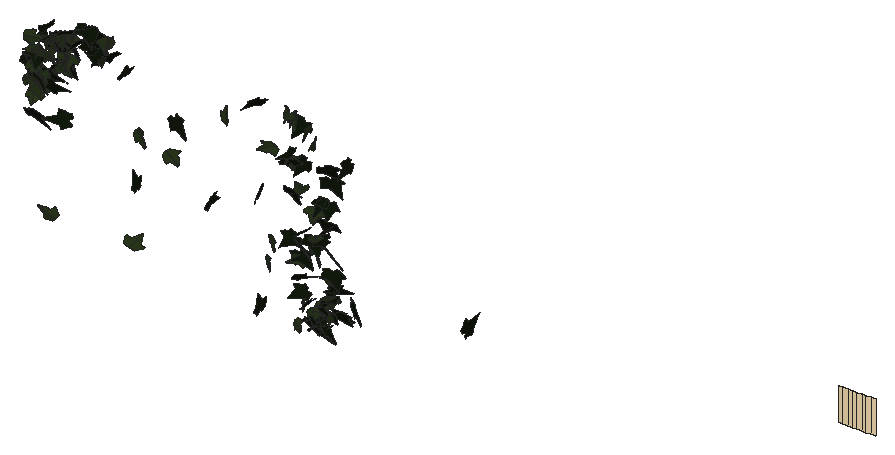
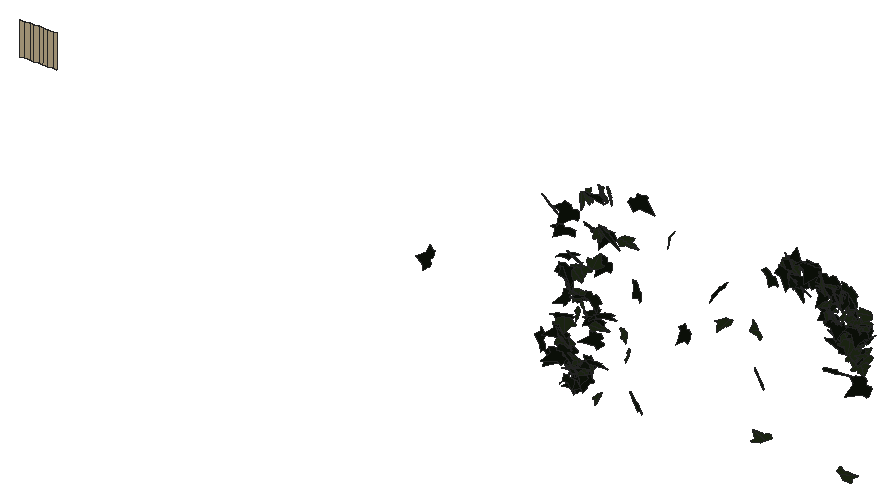
# SketchUp Ruby script. Lengths in inches.
U = 1.inch
M = Sketchup.active_model
def pt(a) = Geom::Point3d.new(a.map { |v| v * U })
def face(e, loops, mat)
  f = e.add_face(loops[0].map { |a| pt(a) })
  loops[1..].each { |l| e.add_face(l.map { |a| pt(a) }).erase! }
  f.material = f.back_material = mat if mat
  f
end
# faces: each face lists its corners as indices into pts; further lists are holes
def faces(e, pts, list, mat = nil) = list.each { |f| face(e, (f[0].is_a?(Array) ? f : [f]).map { |l| l.map { |i| pts[i] } }, mat) }
# xy, xz, yz: faces in a plane at the given z, y or x. An outline is a flat list of corners, or four numbers for a rectangle; further outlines are holes
def ring(l) = l.size == 4 ? [[l[0], l[1]], [l[2], l[1]], [l[2], l[3]], [l[0], l[3]]] : l.each_slice(2).to_a
def flat(e, list, mat, &to3) = list.each { |f| face(e, (f[0].is_a?(Array) ? f : [f]).map { |l| ring(l).map { |u, v| to3.(u, v) } }, mat) }
def xy(e, z, list, mat = nil) = flat(e, list, mat) { |x, y| [x, y, z] }
def xz(e, y, list, mat = nil) = flat(e, list, mat) { |x, z| [x, y, z] }
def yz(e, x, list, mat = nil) = flat(e, list, mat) { |y, z| [x, y, z] }
def lines(e, pts, list) = list.each { |a, b| e.add_line(pt(pts[a]), pt(pts[b])) }
# prism: a flat outline (further loops are holes) pulled along v
def prism(e, loops, v, mat = nil)
  f = face(e, loops, mat); d = Geom::Vector3d.new(v.map { |x| x * U })
  f.pushpull(f.normal.samedirection?(d) ? d.length : -d.length)
end
def box(e, o, s, mat = nil) = prism(e, [[o, [o[0] + s[0], o[1], o[2]], [o[0] + s[0], o[1] + s[1], o[2]], [o[0], o[1] + s[1], o[2]]]], [0, 0, s[2]], mat)
def at(x, y, z, deg = 0) = Geom::Transformation.translation(pt([x, y, z])) * Geom::Transformation.rotation(ORIGIN, Z_AXIS, deg.degrees)
def axes(o, x, y, z) = Geom::Transformation.new([*x, 0, *y, 0, *z, 0, *pt(o).to_a, 1])
def part(name) = M.definitions.add(name)
# library, detail: a bought-in or finely detailed component or shape, given as its bounding box
def library(name, o, s) = part(name).tap { |d| box(d.entities, o, s) }
def detail(e, o, s) = box(e.add_group.entities, o, s)
def put(e, d, t, mat = nil) = e.add_instance(d, t).tap { |i| i.material = mat if mat }
def group(e, t, mat = nil) = e.add_group.tap { |g| g.transformation = t; g.material = mat if mat }.entities
root = M.entities
M.materials.add("1026 AP 7946 SUNNY SIDE UP").color = [254, 231, 186]
M.materials.add("efeu1").color = [18, 25, 13]
M.materials.add("efeu2").color = [43, 57, 29]
c1 = part("ivyleaf_9")
p = [[1.54,2.16,1.25],[1.36,2.04,1.19],[-0.21,0.99,0.68],[-0.71,1.11,0.82],[-0.85,0.86,0.67],[-0.8,0.17,0.21],
  [-0.9,-0.01,0.1],[-0.67,-0.16,-0.02],[-0.08,-0.08,-0.05],[-0.03,-0.6,-0.4],[0.65,-0.88,-0.66],[0.83,-0.6,-0.49],
  [1.29,-0.42,-0.43],[1.8125,-0.07,-0.26],[1.21,0.44,0.15]]
faces(c1.entities,p,[[0,1,2,3,4,5,6,7,8,9,10,11,12,13,14]],"efeu1")
c2 = part("ivyleaf_10")
p = [[0,0.5,-0.03],[-0.0625,2.02,-0.43],[-0.19,2.01,-0.46],[-0.54,1.05,-0.29],[-0.52,0.625,-0.18],[-0.83,0.76,-0.28],
  [-1.16,0.64,-0.33],[-1.15,0.33,-0.24],[-0.77,-0.39,0.02],[-0.3,-0.51,0.16],[0.04,-0.48,0.23],[-0.02,2.01,-0.4375],
  [-0.06,2.01,-0.43],[0.04,-0.49,0.23],[0.67,-0.49,0.14],[1.38,0.36,-0.2],[1.375,0.51,-0.24],[0.81,0.65,-0.19],
  [0.62,0.59,-0.15],[0.6,1.09,-0.28],[0.5,1.23,-0.31]]
faces(c2.entities,p,[[0,1,2,3,4,5,6,7,8,9,10],[11,12,0,13,14,15,16,17,18,19,20]],"efeu2")
xz(root,213,[[177,274,177.27,276]],"1026 AP 7946 SUNNY SIDE UP")
xz(root,213.01,[[177.54,274,177.82,276]],"1026 AP 7946 SUNNY SIDE UP")
p = [[177.54,213.01,276],[177.27,213,276],[177.27,213,274],[177.54,213.01,274],[178.09,213.02,276],[177.82,213.01,276],
  [177.82,213.01,274],[178.09,213.02,274],[178.36,213.04,276],[178.36,213.04,274],[178.63,213.05,276],[178.63,213.05,274],
  [178.9,213.07,276],[178.9,213.07,274],[179.18,213.09,276],[179.18,213.09,274]]
faces(root,p,[[0,1,2,3],[4,5,6,7],[8,4,7,9],[10,8,9,11],[12,10,11,13],[14,12,13,15]],"1026 AP 7946 SUNNY SIDE UP")
put(root,c1,axes([127.72,212.82,276.75],[0.3772,-0.17588,-0.0113],[-0.03293,-0.01175,-0.30568],[0.27503,0.23981,-0.0211]),"1026 AP 7946 SUNNY SIDE UP")
put(root,c1,axes([127.84,212.98,276.51],[-0.03313,-0.29209,0.03896],[-0.00412,-0.03939,-0.30192],[0.46344,-0.02123,0.0001]),"1026 AP 7946 SUNNY SIDE UP")
put(root,c2,axes([127.84,212.9375,275.58],[0.19907,0.21946,0.15502],[0.10288,0.13443,-0.26006],[-0.40443,0.14222,0.01015]),"1026 AP 7946 SUNNY SIDE UP")
put(root,c2,axes([128.36,212.99,275.375],[-0.19765,-0.16137,-0.29884],[-0.3084,-0.21293,0.209],[-0.41954,0.23255,-0.01284]),"1026 AP 7946 SUNNY SIDE UP")
put(root,c2,axes([128.24,212.89,277.32],[-0.28047,-0.24117,0.03904],[0.03255,-0.06335,-0.30437],[0.38282,-0.1713,0.05448]),"1026 AP 7946 SUNNY SIDE UP")
put(root,c2,axes([127.87,212.87,277.85],[0.01117,-0.04427,-0.31213],[0.47775,0.03654,0.00205],[0.05643,-0.3006,0.0444]),"1026 AP 7946 SUNNY SIDE UP")
put(root,c2,axes([128.22,212.84,274.9],[0.26575,0.23024,-0.07491],[-0.06573,-0.06114,-0.29458],[-0.37456,0.17408,-0.00145]),"1026 AP 7946 SUNNY SIDE UP")
put(root,c1,axes([128.29,212.93,276.88],[0.24041,0.25089,-0.02975],[-0.00445,-0.03372,-0.30247],[-0.39734,0.15218,-0.01462]),"1026 AP 7946 SUNNY SIDE UP")
put(root,c2,axes([128.28,212.81,276.48],[0.30804,0.21571,-0.04422],[-0.04426,-0.03407,-0.30038],[-0.34337,0.19791,-0.00095]),"1026 AP 7946 SUNNY SIDE UP")
put(root,c1,axes([128.06,213.05,275.61],[0.33056,-0.19766,0.04801],[0.03066,-0.04874,-0.2967],[0.31826,0.21,-0.02129]),"1026 AP 7946 SUNNY SIDE UP")
put(root,c1,axes([128.11,212.73,273.87],[0.55453,-0.02015,0.01727],[0.0234,-0.03414,-0.36249],[0.03408,0.35141,-0.03215]),"1026 AP 7946 SUNNY SIDE UP")
put(root,c2,axes([128.41,212.91,277.33],[0.1914,-0.27526,-0.02861],[0.00493,0.03001,-0.30951],[0.43476,0.12084,0.01611]),"1026 AP 7946 SUNNY SIDE UP")
put(root,c2,axes([128.42,212.87,277.14],[-0.43618,-0.11328,-0.0391],[0.07091,-0.01219,-0.30739],[0.17361,-0.27963,0.02733]),"1026 AP 7946 SUNNY SIDE UP")
put(root,c1,axes([128.39,212.96,277.1],[-0.24385,-0.25558,-0.01952],[0.07625,-0.00921,-0.30434],[0.39554,-0.15579,0.04664]),"1026 AP 7946 SUNNY SIDE UP")
put(root,c2,axes([128.62,212.82,275.27],[-0.33885,-0.20376,-0.00949],[0.07116,-0.03636,-0.29995],[0.31264,-0.21256,0.05798]),"1026 AP 7946 SUNNY SIDE UP")
put(root,c1,axes([128.42,212.95,275.92],[0.10873,-0.28118,0.05193],[0.00159,-0.05327,-0.29838],[0.44963,0.06819,-0.0115]),"1026 AP 7946 SUNNY SIDE UP")
put(root,c2,axes([128.78,212.875,277.31],[-0.39148,0.15558,0.05274],[-0.08242,0.01087,-0.3018],[-0.24354,-0.25377,0.01736]),"1026 AP 7946 SUNNY SIDE UP")
put(root,c1,axes([128.98,212.83,278.2],[0.09419,-0.01024,-0.31194],[-0.47602,0.0086,-0.06196],[0.01639,0.30849,-0.00682]),"1026 AP 7946 SUNNY SIDE UP")
put(root,c2,axes([128.78,213.05,276.11],[-0.31893,-0.20553,-0.05828],[0.07414,0.03126,-0.29707],[0.32641,-0.20792,0.01052]),"1026 AP 7946 SUNNY SIDE UP")
put(root,c2,axes([128.56,212.9,275.94],[-0.09362,-0.03822,-0.29694],[0.4441,0.06135,-0.06818],[0.10716,-0.28764,0.02312]),"1026 AP 7946 SUNNY SIDE UP")
put(root,c1,axes([129.11,212.68,278.77],[-0.08346,0.29508,0.10232],[-0.08524,0.08876,-0.30614],[-0.48124,-0.06689,0.03648]),"1026 AP 7946 SUNNY SIDE UP")
put(root,c2,axes([129.14,212.74,278.06],[-0.39491,0.13264,0.11658],[-0.17931,0.0234,-0.2908],[-0.20636,-0.27416,0.02959]),"1026 AP 7946 SUNNY SIDE UP")
put(root,c2,axes([129.38,212.8,268.59],[0.20641,0.05303,0.27768],[-0.41919,-0.0461,0.14299],[0.10227,-0.29597,0.02565]),"1026 AP 7946 SUNNY SIDE UP")
put(root,c2,axes([129.125,212.91,276.26],[-0.16047,-0.26226,0.09568],[0.04108,-0.10905,-0.28376],[0.43633,-0.08619,0.0619]),"1026 AP 7946 SUNNY SIDE UP")
put(root,c1,axes([129.25,212.66,278.4],[0.13481,0.28631,0.09483],[0.04095,0.08659,-0.30739],[-0.47033,0.08961,0.00042]),"1026 AP 7946 SUNNY SIDE UP")
put(root,c2,axes([129.26,212.8,277.45],[-0.09505,0.29159,0.03706],[-0.03996,0.02971,-0.30599],[-0.45992,-0.06284,0.01893]),"1026 AP 7946 SUNNY SIDE UP")
put(root,c2,axes([129.34,212.88,278.39],[0.05604,-0.30396,-0.03565],[-0.00996,0.03236,-0.31509],[0.48064,0.03611,-0.00237]),"1026 AP 7946 SUNNY SIDE UP")
put(root,c1,axes([128.95,212.89,276.16],[0.24432,-0.06917,0.25192],[0.32008,-0.13848,-0.17413],[0.24023,0.25487,-0.0242]),"1026 AP 7946 SUNNY SIDE UP")
put(root,c2,axes([129.45,212.8,278.22],[-0.1584,0.28264,0.06675],[-0.06656,0.05181,-0.30798],[-0.4505,-0.10703,0.02203]),"1026 AP 7946 SUNNY SIDE UP")
put(root,c1,axes([129.09,212.83,275.61],[0.21776,-0.03194,0.26995],[0.37102,-0.11815,-0.1439],[0.18675,0.27199,-0.02889]),"1026 AP 7946 SUNNY SIDE UP")
put(root,c1,axes([129.58,212.93,276.82],[0.15077,0.28234,0.00082],[0.02255,-0.00573,-0.3068],[-0.44338,0.09572,-0.01533]),"1026 AP 7946 SUNNY SIDE UP")
put(root,c1,axes([130.12,212.88,278.02],[-0.23549,0.20348,0.17609],[-0.17196,0.13017,-0.25935],[-0.37956,-0.18522,0.00825]),"1026 AP 7946 SUNNY SIDE UP")
put(root,c1,axes([130.2,212.88,274.03],[-0.37111,0.06562,0.1874],[-0.30267,-0.05859,-0.23634],[-0.02267,-0.29193,0.08769]),"1026 AP 7946 SUNNY SIDE UP")
put(root,c1,axes([129.58,212.98,277.93],[0.31187,-0.22627,-0.02112],[0.01989,0.03647,-0.30784],[0.35651,0.1959,0.03564]),"1026 AP 7946 SUNNY SIDE UP")
put(root,c2,axes([129.84,212.91,278.43],[0.19956,-0.26697,0.08135],[0.0486,-0.07442,-0.30493],[0.43574,0.13057,-0.00325]),"1026 AP 7946 SUNNY SIDE UP")
put(root,c1,axes([129.51,212.9,278.18],[0.1997,-0.06727,0.2771],[0.32797,-0.17237,-0.14667],[0.28812,0.24284,-0.0251]),"1026 AP 7946 SUNNY SIDE UP")
put(root,c2,axes([129.78,212.9,277],[0.19238,-0.19906,-0.19635],[0.18736,-0.14846,0.23909],[-0.38938,-0.16978,0.01803]),"1026 AP 7946 SUNNY SIDE UP")
put(root,c2,axes([129.99,212.83,277.72],[0.12334,0.28494,0.05984],[-0.01354,0.06075,-0.3031],[-0.45655,0.07518,0.02516]),"1026 AP 7946 SUNNY SIDE UP")
put(root,c2,axes([129.74,212.89,276.88],[0.24954,0.01367,0.26287],[0.39819,0.03109,-0.16384],[-0.05285,0.29881,0.00679]),"1026 AP 7946 SUNNY SIDE UP")
put(root,c2,axes([130.15,212.88,278.51],[-0.16568,-0.28228,0.06208],[0.006,-0.0672,-0.30958],[0.45434,-0.10204,0.02673]),"1026 AP 7946 SUNNY SIDE UP")
put(root,c2,axes([130,213.03,277.07],[0.44773,-0.07765,0.04491],[0.07586,0.01002,-0.30314],[0.11809,0.28795,0.02447]),"1026 AP 7946 SUNNY SIDE UP")
put(root,c2,axes([130.15,212.79,277.42],[0.10909,-0.27345,-0.10525],[-0.00688,0.10244,-0.28932],[0.4581,0.06665,0.02072]),"1026 AP 7946 SUNNY SIDE UP")
put(root,c2,axes([130.16,212.81,278.57],[-0.37367,-0.18679,-0.06185],[0.11683,-0.00016,-0.30789],[0.28498,-0.24485,0.04512]),"1026 AP 7946 SUNNY SIDE UP")
put(root,c1,axes([130.28,212.73,278.94],[0.15874,0.28628,-0.06325],[-0.05359,-0.05474,-0.31273],[-0.4578,0.10567,0.01468]),"1026 AP 7946 SUNNY SIDE UP")
put(root,c2,axes([130.3,212.91,277.53],[-0.47357,-0.01469,0.02581],[-0.02733,-0.11885,-0.2868],[0.03673,-0.27787,0.11937]),"1026 AP 7946 SUNNY SIDE UP")
put(root,c1,axes([129.99,212.96,277.1875],[-0.14435,-0.07678,-0.28345],[0.38085,0.13143,-0.12046],[0.23688,-0.2581,0.02095]),"1026 AP 7946 SUNNY SIDE UP")
put(root,c2,axes([130.17,212.96,278.64],[0.40143,0.16201,0.01092],[0.02784,-0.00987,-0.31101],[-0.25367,0.25529,-0.01686]),"1026 AP 7946 SUNNY SIDE UP")
put(root,c1,axes([130.41,212.89,278.2],[0.40251,-0.09391,-0.14249],[-0.21722,0.02192,-0.27968],[0.14683,0.28988,-0.02313]),"1026 AP 7946 SUNNY SIDE UP")
put(root,c2,axes([130.42,212.98,278.62],[0.17879,-0.27689,-0.05731],[0.04385,-0.04696,0.30799],[-0.44143,-0.11681,0.00738]),"1026 AP 7946 SUNNY SIDE UP")
put(root,c1,axes([131.08,212.86,278.6875],[-0.16575,0.2283,-0.17618],[0.03456,-0.17664,-0.25597],[-0.44842,-0.098,0.04539]),"1026 AP 7946 SUNNY SIDE UP")
put(root,c1,axes([131.1,212.88,279.29],[0.26798,0.2545,0.05896],[0.07289,0.03598,-0.31477],[-0.40314,0.17568,-0.01772]),"1026 AP 7946 SUNNY SIDE UP")
put(root,c1,axes([131.42,212.96,279.42],[-0.23596,-0.22658,-0.15069],[0.1514,0.10978,-0.27876],[0.39495,-0.17745,0.01683]),"1026 AP 7946 SUNNY SIDE UP")
put(root,c1,axes([131.46,212.9,278.32],[-0.06059,0.01459,0.31302],[0.45376,0.09835,0.03342],[-0.15086,0.28997,-0.02519]),"1026 AP 7946 SUNNY SIDE UP")
put(root,c1,axes([132.22,212.82,278.08],[-0.19198,0.20042,0.20833],[-0.19808,0.15792,-0.24002],[-0.40006,-0.17436,0.01887]),"1026 AP 7946 SUNNY SIDE UP")
put(root,c1,axes([132.26,212.8125,278.08],[-0.12065,0.29944,-0.0002],[-0.00639,-0.00299,-0.31843],[-0.47081,-0.0767,0.00437]),"1026 AP 7946 SUNNY SIDE UP")
put(root,c2,axes([132.42,213.01,279.125],[-0.3998,0.01628,0.17805],[-0.26533,-0.0945,-0.24726],[0.06347,-0.2925,0.0879]),"1026 AP 7946 SUNNY SIDE UP")
put(root,c1,axes([132.29,212.88,278.93],[0.25728,0.14098,0.22892],[-0.29182,-0.12237,0.22084],[0.29187,-0.24662,0.01901]),"1026 AP 7946 SUNNY SIDE UP")
put(root,c2,axes([132.55,212.8125,278.31],[0.05576,-0.30783,-0.01434],[-0.00173,0.01212,-0.31915],[0.4844,0.03548,0.00051]),"1026 AP 7946 SUNNY SIDE UP")
put(root,c2,axes([132.6,212.89,279.23],[-0.27559,-0.25118,0.04992],[0.02558,-0.07125,-0.31111],[0.40186,-0.16772,0.05404]),"1026 AP 7946 SUNNY SIDE UP")
put(root,c1,axes([132.76,212.81,278.48],[0.12967,0.29952,-0.00782],[0.00703,-0.01087,-0.32003],[-0.47115,0.08228,-0.00692]),"1026 AP 7946 SUNNY SIDE UP")
put(root,c2,axes([132.64,212.9,279.24],[0.34883,-0.21175,0.047],[0.06762,-0.0227,-0.31578],[0.33422,0.22559,0.01484]),"1026 AP 7946 SUNNY SIDE UP")
put(root,c1,axes([133.78,212.73,277.83],[0.08933,0.21082,0.23128],[-0.03226,0.22919,-0.21619],[-0.4818,0.02374,0.05736]),"1026 AP 7946 SUNNY SIDE UP")
put(root,c1,axes([134.53,212.75,271.98],[-0.01133,0.08904,0.33242],[-0.08047,0.31815,-0.0899],[-0.51937,-0.05124,0.00668]),"1026 AP 7946 SUNNY SIDE UP")
put(root,c2,axes([134.28,212.71,268.79],[0.32912,0.13796,-0.20637],[0.23478,0.13704,0.25775],[0.3032,-0.25588,0.02442]),"1026 AP 7946 SUNNY SIDE UP")
put(root,c2,axes([134.41,213.02,274.77],[0.24533,-0.09537,0.29509],[0.41343,-0.11677,-0.18792],[0.23493,0.30508,0.02254]),"1026 AP 7946 SUNNY SIDE UP")
put(root,c2,axes([136.46,212.79,274.44],[0.14789,0.27129,0.16515],[0.11423,0.14247,-0.2943],[-0.48088,0.11728,-0.01912]),"1026 AP 7946 SUNNY SIDE UP")
put(root,c1,axes([136.64,213.02,276.3],[0.17637,-0.28511,-0.17208],[-0.12822,0.14529,-0.31411],[0.50218,0.13723,-0.01977]),"1026 AP 7946 SUNNY SIDE UP")
put(root,c1,axes([139.11,212.58,272.91],[-0.06118,0.08433,-0.33385],[-0.2875,0.26854,0.09604],[0.44198,0.18635,0.01626]),"1026 AP 7946 SUNNY SIDE UP")
put(root,c2,axes([140,212.625,277.63],[-0.00525,0.19291,-0.28334],[-0.0527,0.27458,0.19965],[0.52702,0.02938,0.01714]),"1026 AP 7946 SUNNY SIDE UP")
put(root,c1,axes([141.85,212.87,279.23],[-0.13009,0.18799,-0.24589],[-0.03412,-0.25144,-0.19687],[-0.47784,-0.03323,0.081]),"1026 AP 7946 SUNNY SIDE UP")
put(root,c1,axes([142.09,212.66,268.03],[0.00463,0.16662,0.32763],[-0.06497,0.31514,-0.16836],[-0.55947,-0.03522,0.02226]),"1026 AP 7946 SUNNY SIDE UP")
put(root,c1,axes([141.99,212.6,274.11],[0.02629,0.13967,0.32731],[0.08537,0.31231,-0.14292],[-0.53784,0.0564,-0.00669]),"1026 AP 7946 SUNNY SIDE UP")
put(root,c2,axes([142.51,213.03,276.875],[0.27788,0.02154,-0.24451],[-0.37268,-0.01641,-0.18334],[-0.04094,0.29555,0.00938]),"1026 AP 7946 SUNNY SIDE UP")
put(root,c2,axes([142.34,212.9,270.71],[-0.14511,0.26128,0.01232],[-0.0246,0.00557,-0.28512],[-0.41043,-0.09271,0.01274]),"1026 AP 7946 SUNNY SIDE UP")
put(root,c2,axes([142.4,213.11,271.82],[-0.2497,0.1734,-0.15429],[0.09789,-0.14392,-0.23896],[-0.34778,-0.16502,0.04352]),"1026 AP 7946 SUNNY SIDE UP")
put(root,c2,axes([143.54,212.92,279.11],[0.11874,-0.20713,-0.2351],[-0.15157,0.20603,-0.22547],[0.45885,0.12165,-0.01364]),"1026 AP 7946 SUNNY SIDE UP")
put(root,c1,axes([143.74,212.98,276.89],[-0.3078,0.23665,0.01523],[-0.03535,-0.00119,-0.31585],[-0.37103,-0.19621,0.01746]),"1026 AP 7946 SUNNY SIDE UP")
put(root,c1,axes([143.82,213.14,272.37],[-0.36189,-0.13626,0.07683],[-0.08249,-0.05874,-0.27487],[0.23052,-0.23494,0.02224]),"1026 AP 7946 SUNNY SIDE UP")
put(root,c2,axes([143.84,213.08,279.05],[0.22137,-0.27343,0.07841],[0.04504,-0.07258,-0.31716],[0.44467,0.14347,-0.00691]),"1026 AP 7946 SUNNY SIDE UP")
put(root,c1,axes([143.8,212.71,276.68],[0.36127,0.18226,-0.04889],[-0.03766,-0.04761,-0.30154],[-0.29415,0.22994,-0.02144]),"1026 AP 7946 SUNNY SIDE UP")
put(root,c1,axes([143.79,212.78,275.08],[0.4478,-0.02191,-0.08184],[-0.12731,-0.02372,-0.29289],[0.02304,0.29467,-0.02791]),"1026 AP 7946 SUNNY SIDE UP")
put(root,c2,axes([144.04,213.01,276.76],[-0.19191,-0.265,0.08528],[0.00558,-0.09352,-0.29818],[0.43722,-0.11513,0.04124]),"1026 AP 7946 SUNNY SIDE UP")
put(root,c2,axes([143.77,213.07,278.98],[0.31864,-0.12528,0.20888],[0.26086,-0.11824,-0.24591],[0.27041,0.2617,-0.00891]),"1026 AP 7946 SUNNY SIDE UP")
put(root,c2,axes([144.18,213.21,274.98],[-0.22496,-0.20454,-0.15601],[-0.16168,-0.11101,0.25585],[-0.36488,0.1753,-0.01718]),"1026 AP 7946 SUNNY SIDE UP")
put(root,c2,axes([144.06,213,267.85],[0.01089,0.24784,0.06067],[-0.02315,0.0578,-0.25455],[-0.39937,0.00341,0.01641]),"1026 AP 7946 SUNNY SIDE UP")
put(root,c2,axes([144.4,212.88,271.48],[0.20417,0.0464,-0.23794],[-0.3343,-0.09123,-0.14238],[-0.16053,0.24901,-0.00612]),"1026 AP 7946 SUNNY SIDE UP")
put(root,c1,axes([144.34,213.18,278.75],[-0.4419,-0.11596,-0.04247],[0.08331,-0.02302,-0.31046],[0.17429,-0.28301,0.04071]),"1026 AP 7946 SUNNY SIDE UP")
put(root,c1,axes([144.47,213.17,269.62],[-0.38281,-0.03663,0.07555],[-0.10693,-0.03922,-0.25228],[0.07249,-0.25128,0.02683]),"1026 AP 7946 SUNNY SIDE UP")
put(root,c1,axes([144.54,212.83,273],[0.00787,0.27018,0.05762],[-0.04925,0.05461,-0.27614],[-0.43054,-0.00131,0.03264]),"1026 AP 7946 SUNNY SIDE UP")
put(root,c1,axes([144.62,212.97,276.8125],[-0.44066,0.01224,-0.10049],[0.15091,-0.03075,-0.28801],[-0.034,-0.29516,0.02409]),"1026 AP 7946 SUNNY SIDE UP")
put(root,c2,axes([144.64,212.76,269.2],[-0.09292,0.20811,0.1556],[-0.18002,0.1162,-0.21208],[-0.36084,-0.11156,0.06574]),"1026 AP 7946 SUNNY SIDE UP")
put(root,c1,axes([144.3,212.98,272.14],[0.18127,-0.21057,0.13125],[0.1025,-0.11091,-0.24793],[0.37417,0.13239,0.00433]),"1026 AP 7946 SUNNY SIDE UP")
put(root,c1,axes([144.32,212.66,270.57],[0.28843,0.04825,0.20662],[0.25435,0.13236,-0.18468],[-0.20063,0.23716,0.06291]),"1026 AP 7946 SUNNY SIDE UP")
put(root,c1,axes([144.35,212.91,271.8],[-0.10306,-0.15223,-0.23192],[0.24818,0.16613,-0.16273],[0.34648,-0.16428,0.04758]),"1026 AP 7946 SUNNY SIDE UP")
put(root,c2,axes([144.7,213.08,278.5625],[0.1238,-0.22967,0.20424],[0.09142,-0.19098,-0.25118],[0.4696,0.09773,-0.00494]),"1026 AP 7946 SUNNY SIDE UP")
put(root,c1,axes([144.79,212.65,269.18],[0.13971,0.11119,0.23095],[0.145,0.20589,-0.14205],[-0.36483,0.12441,0.03198]),"1026 AP 7946 SUNNY SIDE UP")
put(root,c2,axes([145.12,212.91,272.32],[-0.03093,0.15045,0.24146],[-0.32594,0.14791,-0.11529],[-0.29081,-0.18178,0.10354]),"1026 AP 7946 SUNNY SIDE UP")
put(root,c2,axes([145.05,213.02,268.8125],[0.14528,0.16671,-0.16633],[-0.10843,-0.14727,-0.19703],[-0.34952,0.11498,-0.00801]),"1026 AP 7946 SUNNY SIDE UP")
put(root,c1,axes([145.07,212.83,268.46],[0.25965,0.17244,-0.09338],[-0.07393,-0.08135,-0.2455],[-0.298,0.17043,-0.02046]),"1026 AP 7946 SUNNY SIDE UP")
put(root,c1,axes([145.12,212.74,268.67],[0.11104,0.23281,0.09539],[0.05455,0.0848,-0.24999],[-0.38939,0.07827,-0.00782]),"1026 AP 7946 SUNNY SIDE UP")
put(root,c2,axes([145.27,212.78,278.18],[0.04472,-0.28487,-0.12241],[0.02117,0.11874,-0.29326],[0.4839,0.02113,0.02414]),"1026 AP 7946 SUNNY SIDE UP")
put(root,c2,axes([145.18,212.9,274.4],[0.44331,0.06615,-0.00111],[0.00707,-0.0255,-0.29729],[-0.1038,0.28078,-0.02499]),"1026 AP 7946 SUNNY SIDE UP")
put(root,c1,axes([145.24,212.75,268.12],[0.16572,0.17716,0.15475],[0.10732,0.1329,-0.21145],[-0.34803,0.12534,0.00848]),"1026 AP 7946 SUNNY SIDE UP")
put(root,c2,axes([145.36,213.14,274.15],[-0.06422,-0.25089,0.13841],[-0.01198,-0.13615,-0.26234],[0.44841,-0.03957,0.01281]),"1026 AP 7946 SUNNY SIDE UP")
put(root,c1,axes([145.18,212.91,272.82],[-0.15121,-0.24371,-0.10501],[0.12206,0.07611,-0.26609],[0.39618,-0.11647,0.0419]),"1026 AP 7946 SUNNY SIDE UP")
put(root,c1,axes([145.22,212.8,268.63],[0.21387,-0.18118,-0.12887],[-0.13937,0.08822,-0.23231],[0.3159,0.16158,-0.01525]),"1026 AP 7946 SUNNY SIDE UP")
put(root,c2,axes([145.35,212.95,271.92],[-0.23541,0.23072,0.00436],[-0.029,-0.00849,-0.28264],[-0.36166,-0.1495,0.01983]),"1026 AP 7946 SUNNY SIDE UP")
put(root,c2,axes([145.35,212.86,272.94],[-0.36157,-0.13339,-0.09893],[0.16773,0.00284,-0.26933],[0.1957,-0.24889,0.04807]),"1026 AP 7946 SUNNY SIDE UP")
put(root,c1,axes([145.57,213.09,274.93],[-0.37835,-0.03429,-0.16761],[0.25667,-0.10163,-0.2275],[-0.0482,-0.27199,0.10429]),"1026 AP 7946 SUNNY SIDE UP")
put(root,c2,axes([145.41,212.8,269.01],[-0.04849,-0.10697,-0.2493],[0.28433,0.16853,-0.09975],[0.30251,-0.17555,0.05379]),"1026 AP 7946 SUNNY SIDE UP")
put(root,c1,axes([145.32,212.91,267.93],[0.34516,-0.0865,0.10519],[0.13552,-0.0599,-0.24234],[0.16173,0.23479,-0.02142]),"1026 AP 7946 SUNNY SIDE UP")
put(root,c1,axes([145.83,212.89,268.82],[-0.23753,0.19114,-0.07765],[0.02262,-0.0848,-0.24818],[-0.32291,-0.14654,0.03973]),"1026 AP 7946 SUNNY SIDE UP")
put(root,c1,axes([145.65,213.18,268.87],[-0.224,-0.21214,0.01126],[0.10963,-0.06047,-0.24616],[0.31562,-0.12956,0.09349]),"1026 AP 7946 SUNNY SIDE UP")
put(root,c1,axes([145.96,212.86,273.06],[-0.37808,0.13792,-0.04223],[-0.00137,-0.08266,-0.27643],[-0.22659,-0.22962,0.07214]),"1026 AP 7946 SUNNY SIDE UP")
put(root,c1,axes([145.86,212.94,268.11],[-0.01725,0.25011,0.01715],[-0.01227,0.01489,-0.25771],[-0.3938,-0.01142,0.00728]),"1026 AP 7946 SUNNY SIDE UP")
put(root,c2,axes([145.62,213,269.39],[0.37836,-0.00439,0.10215],[0.15492,-0.02146,-0.24735],[0.01922,0.25938,-0.01721]),"1026 AP 7946 SUNNY SIDE UP")
put(root,c1,axes([146.02,212.83,269.16],[0.29324,0.06157,-0.26113],[-0.36128,-0.10966,-0.20194],[-0.19532,0.29527,-0.01851]),"1026 AP 7946 SUNNY SIDE UP")
put(root,c1,axes([146.06,212.82,274.03],[0.31671,0.13521,-0.18887],[-0.26183,-0.08111,-0.24952],[-0.24587,0.26055,0.02242]),"1026 AP 7946 SUNNY SIDE UP")
put(root,c1,axes([145.92,213.14,274.94],[-0.21648,-0.25514,-0.0286],[0.07058,0.00543,-0.29622],[0.39708,-0.14006,0.03706]),"1026 AP 7946 SUNNY SIDE UP")
put(root,c1,axes([146.14,212.79,269.71],[0.0736,0.28323,-0.04216],[-0.07358,-0.03495,-0.29305],[-0.44429,0.05271,0.04155]),"1026 AP 7946 SUNNY SIDE UP")
put(root,c1,axes([146.15,212.75,273.76],[-0.01886,0.30309,-0.00027],[0.00411,-0.00188,-0.31248],[-0.47656,-0.01201,-0.00268]),"1026 AP 7946 SUNNY SIDE UP")
put(root,c2,axes([146.08,212.86,269.11],[-0.33813,0.18668,0.01119],[-0.05722,-0.02715,-0.28994],[-0.28831,-0.21354,0.04442]),"1026 AP 7946 SUNNY SIDE UP")
put(root,c1,axes([145.95,212.84,268.28],[0.23266,-0.20826,-0.09194],[-0.0851,0.06956,-0.26275],[0.34521,0.15751,-0.00281]),"1026 AP 7946 SUNNY SIDE UP")
put(root,c1,axes([146.39,212.89,270.4],[-0.17107,0.2561,0.08459],[-0.05849,0.07181,-0.28616],[-0.41811,-0.11483,0.00542]),"1026 AP 7946 SUNNY SIDE UP")
put(root,c1,axes([146.04,212.65,277.09],[0.402,0.19432,0.02948],[0.06663,-0.01053,-0.32903],[-0.30132,0.25692,-0.03342]),"1026 AP 7946 SUNNY SIDE UP")
put(root,c1,axes([146.4,212.94,270.14],[-0.41785,0.09401,-0.04809],[0.05145,-0.04804,-0.28856],[-0.15721,-0.26559,0.03337]),"1026 AP 7946 SUNNY SIDE UP")
put(root,c2,axes([146.26,212.89,271.11],[-0.38603,-0.14874,0.00959],[0.00554,-0.02535,-0.29487],[0.23435,-0.2444,0.02278]),"1026 AP 7946 SUNNY SIDE UP")
put(root,c2,axes([146.32,212.875,269.98],[-0.35006,-0.16839,0.00806],[0.00931,-0.02233,-0.28685],[0.26497,-0.22168,0.02072]),"1026 AP 7946 SUNNY SIDE UP")
put(root,c1,axes([146.08,213.0625,276.28],[-0.15633,-0.15662,-0.24858],[0.23146,0.19055,-0.18948],[0.38725,-0.17712,0.01291]),"1026 AP 7946 SUNNY SIDE UP")
put(root,c1,axes([146.04,212.875,272.46],[0.36556,-0.18794,0.00755],[-0.00442,-0.01681,-0.30769],[0.29578,0.23203,-0.01393]),"1026 AP 7946 SUNNY SIDE UP")
put(root,c1,axes([146.36,212.9,271.4],[-0.15956,-0.23844,-0.13096],[0.17913,0.08387,-0.258],[0.38418,-0.13814,0.0659]),"1026 AP 7946 SUNNY SIDE UP")
put(root,c1,axes([146.3,212.87,270.48],[0.31376,0.09412,0.19541],[0.27341,0.07462,-0.22679],[-0.18869,0.26462,-0.00368]),"1026 AP 7946 SUNNY SIDE UP")
put(root,c1,axes([146.375,212.99,269.21],[0.40264,0.02675,0.09484],[0.14414,0.00706,-0.26518],[-0.04334,0.27197,-0.00084]),"1026 AP 7946 SUNNY SIDE UP")
put(root,c1,axes([146.58,212.98,269.16],[0.41458,0.08705,0.01634],[0.03642,-0.02138,-0.28476],[-0.13415,0.26324,-0.02681]),"1026 AP 7946 SUNNY SIDE UP")
put(root,c1,axes([147.17,213.12,277.48],[-0.41949,0.08081,-0.16524],[0.22112,-0.086,-0.28527],[-0.17672,-0.29942,0.03531]),"1026 AP 7946 SUNNY SIDE UP")
put(root,c1,axes([147.29,213.21,269.84],[0.07155,-0.04472,-0.3872],[0.56809,-0.10688,0.05757],[-0.17612,-0.36293,0.02842]),"1026 AP 7946 SUNNY SIDE UP")
put(root,c1,axes([154.72,212.54,271.3],[-0.04032,0.00351,0.40859],[0.34594,0.33079,0.01357],[-0.51888,0.22027,-0.0227]),"1026 AP 7946 SUNNY SIDE UP")
